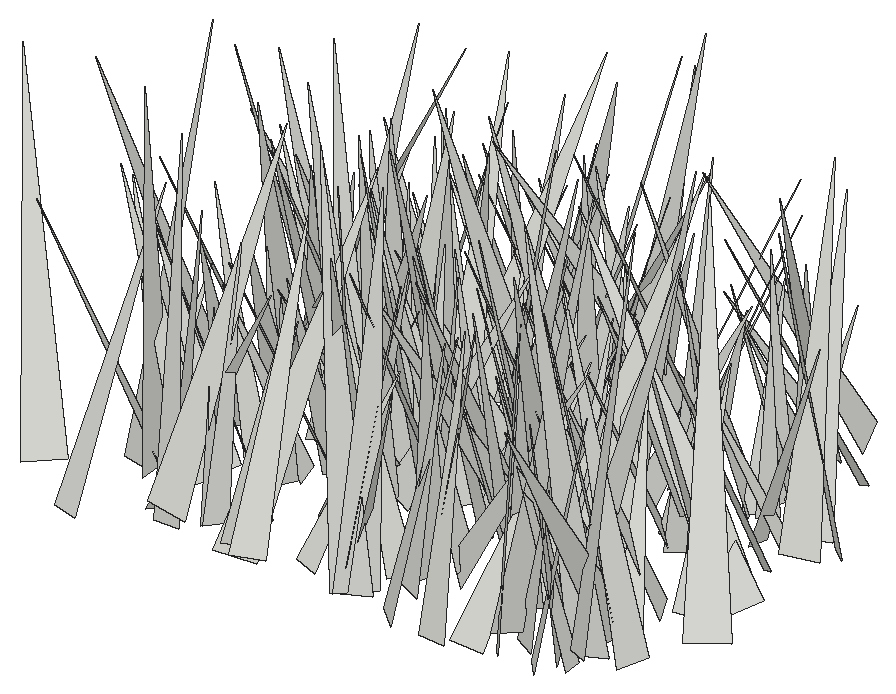
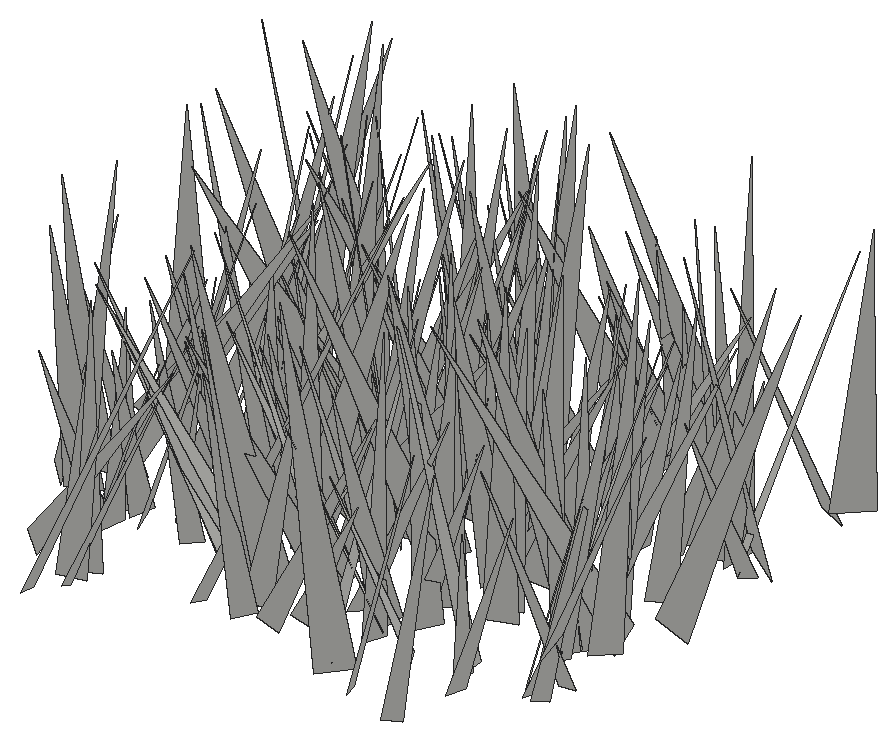
# SketchUp Ruby script. Lengths in inches.
U = 1.inch
M = Sketchup.active_model
def pt(a) = Geom::Point3d.new(a.map { |v| v * U })
def face(e, loops, mat)
  f = e.add_face(loops[0].map { |a| pt(a) })
  loops[1..].each { |l| e.add_face(l.map { |a| pt(a) }).erase! }
  f.material = f.back_material = mat if mat
  f
end
# faces: each face lists its corners as indices into pts; further lists are holes
def faces(e, pts, list, mat = nil) = list.each { |f| face(e, (f[0].is_a?(Array) ? f : [f]).map { |l| l.map { |i| pts[i] } }, mat) }
# xy, xz, yz: faces in a plane at the given z, y or x. An outline is a flat list of corners, or four numbers for a rectangle; further outlines are holes
def ring(l) = l.size == 4 ? [[l[0], l[1]], [l[2], l[1]], [l[2], l[3]], [l[0], l[3]]] : l.each_slice(2).to_a
def flat(e, list, mat, &to3) = list.each { |f| face(e, (f[0].is_a?(Array) ? f : [f]).map { |l| ring(l).map { |u, v| to3.(u, v) } }, mat) }
def xy(e, z, list, mat = nil) = flat(e, list, mat) { |x, y| [x, y, z] }
def xz(e, y, list, mat = nil) = flat(e, list, mat) { |x, z| [x, y, z] }
def yz(e, x, list, mat = nil) = flat(e, list, mat) { |y, z| [x, y, z] }
def lines(e, pts, list) = list.each { |a, b| e.add_line(pt(pts[a]), pt(pts[b])) }
# prism: a flat outline (further loops are holes) pulled along v
def prism(e, loops, v, mat = nil)
  f = face(e, loops, mat); d = Geom::Vector3d.new(v.map { |x| x * U })
  f.pushpull(f.normal.samedirection?(d) ? d.length : -d.length)
end
def box(e, o, s, mat = nil) = prism(e, [[o, [o[0] + s[0], o[1], o[2]], [o[0] + s[0], o[1] + s[1], o[2]], [o[0], o[1] + s[1], o[2]]]], [0, 0, s[2]], mat)
def at(x, y, z, deg = 0) = Geom::Transformation.translation(pt([x, y, z])) * Geom::Transformation.rotation(ORIGIN, Z_AXIS, deg.degrees)
def axes(o, x, y, z) = Geom::Transformation.new([*x, 0, *y, 0, *z, 0, *pt(o).to_a, 1])
def part(name) = M.definitions.add(name)
# library, detail: a bought-in or finely detailed component or shape, given as its bounding box
def library(name, o, s) = part(name).tap { |d| box(d.entities, o, s) }
def detail(e, o, s) = box(e.add_group.entities, o, s)
def put(e, d, t, mat = nil) = e.add_instance(d, t).tap { |i| i.material = mat if mat }
def group(e, t, mat = nil) = e.add_group.tap { |g| g.transformation = t; g.material = mat if mat }.entities
root = M.entities
c1 = part("fur_instance\#9")
p = [[0.8125,0,1.79],[0.67,-0.02,1.48],[0,-0.11,0],[0,0.11,0]]
faces(c1.entities,p,[[0,1,2,3]])
put(root,c1,axes([88.02,156.51,-28.22],[4.64507,-4.79979,0.2726],[-4.36308,-4.36804,-2.56373],[-2.01887,-1.6035,6.16782]))
put(root,c1,axes([77.79,154.35,-28.22],[5.21952,0.68023,0.61562],[0.83808,-4.98198,-1.60081],[-0.37326,-1.674,5.01433]))
put(root,c1,axes([80.74,152.42,-28.22],[3.65147,4.43575,1.22236],[4.5601,-3.69672,-0.20725],[-0.61278,-1.07778,5.74161]))
put(root,c1,axes([81.4,152.85,-27.1],[1.95636,4.4496,1.57567],[4.70552,-1.97342,-0.26957],[-0.3738,-1.55425,4.8532]))
put(root,c1,axes([72.83,152.17,-27.1],[-3.84179,0.25674,0.88435],[-0.00822,3.78425,-1.13434],[0.92083,1.10494,3.67947]))
put(root,c1,axes([82.99,152.11,-28.22],[0.82489,5.68831,1.342],[5.81529,-0.93413,0.38496],[-0.58339,-1.2684,5.73491]))
put(root,c1,axes([87.29,153.95,-28.22],[3.95748,1.9361,2.48086],[2.44941,-4.39763,-0.47534],[-1.97573,-1.57388,4.37997]))
put(root,c1,axes([86.67,151.25,-27.1],[3.82585,4.29132,1.89582],[3.55577,-4.24822,2.44044],[-3.06039,0.42878,5.20545]))
put(root,c1,axes([85.82,153.8125,-28.22],[-0.58036,-3.55618,1.37675],[-3.59236,0.97706,1.00942],[1.27936,1.13031,3.45894]))
put(root,c1,axes([74.38,151.53,-27.1],[-4.08665,1.67614,0.95166],[1.15635,3.91687,-1.93308],[1.54207,1.50482,3.97156]))
put(root,c1,axes([74.78,151.58,-27.1],[2.09645,3.63188,0.13416],[3.39461,-2.01213,1.42535],[-1.29816,0.60366,3.94386]))
put(root,c1,axes([73.05,152.36,-27.1],[-4.76791,1.69378,1.39092],[1.4281,4.92716,-1.10462],[1.66255,0.62512,4.93778]))
put(root,c1,axes([87.03,152.81,-28.22],[3.56693,3.32971,1.1246],[3.34181,-3.70943,0.38354],[-1.08812,-0.47732,4.86445]))
put(root,c1,axes([69.54,153.64,-28.22],[5.28703,-2.12696,0.17156],[-2.11759,-5.17319,1.12251],[0.26309,1.10465,5.58719]))
put(root,c1,axes([81.67,153.56,-28.22],[5.42096,2.25752,1.64956],[2.38588,-5.61122,-0.16143],[-1.45775,-0.7887,5.87002]))
put(root,c1,axes([67.07,151.28,-28.22],[2.05142,5.93925,0.09208],[5.90467,-2.04959,0.65232],[-0.64654,0.12643,6.2496]))
put(root,c1,axes([65.43,152.15,-27.1],[-5.44191,5.3364,0.6963],[5.36336,5.45938,0.07682],[0.44311,-0.54257,7.6214]))
put(root,c1,axes([75.4375,151.14,-27.1],[-4.827,3.94667,0.05385],[3.76525,4.62978,-1.80751],[1.18405,1.36675,5.96733]))
put(root,c1,axes([88.11,153.6875,-28.22],[-5.31837,-1.43549,0.4315],[-1.49067,5.23198,-0.96754],[0.15722,1.04767,5.42306]))
put(root,c1,axes([71.1,151.98,-27.1],[0.33819,7.69063,1.05021],[7.70297,-0.20312,-0.99305],[0.95553,-1.08446,7.63374]))
put(root,c1,axes([67.31,156.37,-28.22],[-4.61159,-4.4726,0.38091],[-4.39573,4.61032,0.9157],[0.90928,-0.396,6.35865]))
put(root,c1,axes([78.73,153.17,-28.22],[-5.99811,4.4385,2.51735],[4.45899,6.44808,-0.74453],[2.48087,-0.8583,7.4245]))
put(root,c1,axes([78.72,152.91,-28.22],[-1.50956,7.97784,1.83345],[8.07703,1.14872,1.65178],[-1.3301,-2.07864,7.94961]))
put(root,c1,axes([78.3125,153.09,-27.1],[3.87453,3.49507,1.24049],[3.40824,-4.0629,0.80191],[-1.46226,-0.20898,5.15601]))
put(root,c1,axes([84.18,155.85,-28.22],[4.37125,-4.19897,0.80164],[-4.19734,-4.43318,-0.33332],[-0.81017,0.31203,6.05212]))
put(root,c1,axes([80.11,155.66,-28.22],[5.51508,-3.1001,1.56666],[-3.03836,-5.73026,-0.64316],[-1.68328,0.18611,6.29389]))
put(root,c1,axes([70.46,152.79,-28.22],[1.63726,6.8228,1.57078],[6.72877,-1.9791,1.58281],[-1.9343,-1.10957,6.83563]))
put(root,c1,axes([76.18,153.52,-28.22],[0.4921,4.23207,0.57816],[4.10963,-0.31046,-1.22532],[1.16432,-0.69285,4.08059]))
put(root,c1,axes([84.22,152.52,-28.22],[-2.22642,5.28944,0.76409],[4.89566,2.35054,-2.00661],[2.14349,0.12554,5.37668]))
put(root,c1,axes([68.81,155.51,-28.22],[3.49606,4.56093,2.47636],[5.16488,-3.35013,-1.12142],[-0.50841,-2.67048,5.63622]))
put(root,c1,axes([88.66,155.73,-28.22],[-5.18557,-4.32883,1.54546],[-4.49087,5.26797,-0.31293],[0.97941,1.23577,6.74766]))
put(root,c1,axes([88.07,154.65,-28.22],[-0.9931,7.68396,2.84346],[8.04191,0.36629,1.81887],[-1.56723,-2.98953,7.53135]))
put(root,c1,axes([79.22,155.12,-28.22],[-4.02277,2.62654,1.01722],[2.78428,3.97624,0.74391],[0.42575,-1.18612,4.74637]))
put(root,c1,axes([88.92,152.92,-27.1],[4.06044,6.49572,1.60929],[6.19974,-4.35997,1.95581],[-2.5194,-0.26008,7.4065]))
put(root,c1,axes([67.64,155.83,-28.22],[7.3985,0.06507,3.2704],[0.28828,-8.06925,-0.49163],[-3.25831,-0.56619,7.38244]))
put(root,c1,axes([85.96,152.64,-27.1],[7.23662,0.86237,3.59764],[-0.54989,-7.56504,2.91946],[-3.65846,2.84288,6.67751]))
put(root,c1,axes([73.79,152.48,-28.22],[-4.61251,5.93847,1.25396],[5.3205,4.71401,-2.75381],[2.92064,0.79104,6.99694]))
put(root,c1,axes([74.57,158.52,-28.22],[5.93446,-4.51627,0.11992],[-4.41947,-5.84426,-1.3935],[-0.93776,-1.03771,7.32616]))
put(root,c1,axes([73.16,155.4,-28.22],[-4.82792,-3.85999,0.34861],[-3.62589,4.30173,-2.58417],[-1.36894,2.21934,5.6152]))
put(root,c1,axes([69.51,155.82,-28.22],[-5.5849,2.54638,0.93821],[2.66389,5.55377,0.78405],[0.51763,-1.10771,6.08773]))
put(root,c1,axes([80.58,156.55,-28.22],[4.45492,4.83666,0.95124],[4.56601,-3.56591,-3.25273],[1.85733,-2.83468,5.71483]))
put(root,c1,axes([89.59,155.23,-28.22],[-6.93734,1.12272,0.61983],[1.08478,6.95591,-0.45824],[0.68406,0.3553,7.01265]))
put(root,c1,axes([85.91,155.92,-28.22],[-6.46812,-3.13785,1.21731],[-3.3431,6.29489,-1.53709],[0.38946,1.92167,7.02282]))
put(root,c1,axes([78.05,159.51,-28.22],[-2.99336,-6.46525,0.18966],[-6.30073,2.9619,1.52434],[1.46161,-0.47255,6.9596]))
put(root,c1,axes([76.05,156.49,-28.22],[-5.53367,-3.1899,2.46645],[-3.58117,5.81278,-0.51687],[1.85312,1.70777,6.3663]))
put(root,c1,axes([82.53,157.33,-28.22],[-3.26871,-2.2439,0.63682],[-2.29753,3.28654,-0.21245],[0.40248,0.53729,3.95909]))
put(root,c1,axes([75.91,156.9,-28.22],[-1.49797,-4.88201,2.75569],[-5.27998,2.18724,1.00478],[1.88406,2.24805,5.00683]))
put(root,c1,axes([71.89,157.7,-28.22],[3.44775,-2.42349,1.09947],[-2.43313,-3.5995,-0.30427],[-1.07797,0.37336,4.2033]))
put(root,c1,axes([82.2,157.69,-28.22],[-1.33118,-5.02308,1.66852],[-5.29255,1.28443,-0.35575],[0.06525,1.70478,5.18429]))
put(root,c1,axes([82.14,159.96,-28.22],[7.22069,-3.00234,1.05262],[-2.62839,-7.10035,-2.22196],[-1.79266,-1.6827,7.49769]))
put(root,c1,axes([88.01,158.9375,-28.22],[-5.06216,-2.56794,0.53616],[-2.44101,5.03776,1.08155],[0.96086,-0.73072,5.57226]))
put(root,c1,axes([85.05,157.84,-28.22],[3.34183,1.38887,0.77255],[1.56239,-3.2005,-1.00466],[-0.29109,-1.23347,3.4767]))
put(root,c1,axes([69.7,157.1875,-28.22],[-4.93751,1.50851,0.32737],[1.53378,4.91815,0.47027],[0.1741,-0.54591,5.14135]))
put(root,c1,axes([68.08,156.23,-28.22],[-3.43494,4.07646,0.13435],[4.04677,3.38429,0.77755],[-0.50915,-0.60283,5.27368]))
put(root,c1,axes([72.09,158.7,-28.22],[-4.26767,-0.91045,0.71231],[-0.70932,4.21373,1.13607],[0.91278,-0.98229,4.21323]))
put(root,c1,axes([81.26,160.03,-28.22],[1.60402,-6.13136,0.73735],[-5.58582,-1.76536,-2.52831],[-2.63361,0.00991,5.81155]))
put(root,c1,axes([80.69,156.97,-28.22],[-7.05105,-1.29004,0.36767],[-1.33665,6.92247,-1.34515],[0.11284,1.38992,7.04075]))
put(root,c1,axes([66.62,156.59,-28.22],[-0.81178,3.59213,0.55552],[3.51446,0.92094,-0.81938],[0.92765,-0.34562,3.5904]))
put(root,c1,axes([86.65,158.11,-28.22],[-4.9499,-5.12629,0.49866],[-4.98162,4.58947,-2.26921],[-1.30806,1.92014,6.75508]))
put(root,c1,axes([86.39,155.75,-28.22],[6.67924,-1.26552,2.75336],[-2.18749,-6.62541,2.26131],[-2.097,2.88046,6.41095]))
put(root,c1,axes([72.96,159.35,-28.22],[1.69834,-4.62751,0.65795],[-4.61755,-1.76962,-0.52709],[-0.72459,0.43091,4.90106]))
put(root,c1,axes([67.92,159.87,-28.22],[3.84252,-3.67557,0.42443],[-3.56655,-3.84235,-0.9854],[-0.98471,-0.42605,5.2253]))
put(root,c1,axes([77.59,158.73,-28.22],[-6.16765,-3.82155,1.90605],[-3.98751,6.35208,-0.16723],[1.52874,1.15063,7.2537]))
put(root,c1,axes([82.94,158.13,-28.22],[-3.53133,-2.30027,1.49102],[-2.55807,3.63918,-0.44418],[0.98523,1.20406,4.19097]))
put(root,c1,axes([73.27,158.94,-28.22],[-3.04212,-3.44962,0.11938],[-3.35963,2.92271,-1.15727],[-0.79185,0.85236,4.45141]))
put(root,c1,axes([66.77,155.62,-28.22],[3.59561,7.30217,1.1805],[7.09033,-3.77639,1.76345],[-2.10771,-0.24675,7.94609]))
put(root,c1,axes([74.57,158.67,-28.22],[1.59006,-7.38899,3.46765],[-7.94346,-2.21328,-1.07372],[-1.87702,3.10714,7.48148]))
put(root,c1,axes([70.87,157.58,-28.22],[-5.26641,1.25593,0.32091],[1.22212,5.2582,-0.5227],[0.43216,0.43524,5.3888]))
put(root,c1,axes([87.9375,157.125,-28.22],[-2.52047,3.62206,0.22803],[3.61381,2.53037,-0.24846],[0.33426,-0.04477,4.40572]))
put(root,c1,axes([74.17,156.91,-28.22],[4.05537,2.07279,0.17475],[1.9711,-3.95155,1.12829],[-0.66463,0.92835,4.41242]))
put(root,c1,axes([75.57,158.63,-28.22],[-6.94561,0.7265,2.56424],[0.79665,7.39636,0.06233],[2.54332,-0.33278,6.98322]))
put(root,c1,axes([84.43,157.01,-28.22],[1.79845,4.31058,0.12569],[4.2592,-1.79684,0.67963],[-0.67534,0.14702,4.621]))
put(root,c1,axes([80.375,160.66,-28.22],[-0.3519,-5.66898,0.64957],[-5.59847,0.21723,-1.13712],[-1.1029,0.70611,5.5649]))
put(root,c1,axes([78.21,158.375,-28.22],[2.39277,4.07076,1.54907],[4.21231,-2.6123,0.35825],[-1.10775,-1.14055,4.7083]))
put(root,c1,axes([75.8,159.96,-28.22],[-1.49578,-4.28811,0.26565],[-3.87905,1.22698,-2.03551],[-1.84701,0.89578,4.0598]))
put(root,c1,axes([84.61,163.27,-28.22],[-3.72735,-5.65721,0.3773],[-4.71825,3.34531,3.54775],[3.14396,-1.68653,5.77153]))
put(root,c1,axes([79.78,159.2,-28.22],[-2.85535,-4.62994,1.75531],[-4.89429,2.33192,-1.81068],[-0.75056,2.40755,5.12941]))
put(root,c1,axes([68.59,161.71,-28.22],[4.17409,-3.35782,0.27535],[-3.2273,-4.11088,-1.20788],[-0.96712,-0.77425,5.2191]))
put(root,c1,axes([77.39,161.27,-28.22],[0.67121,-5.58126,0.90748],[-5.6399,-0.72653,-0.2969],[-0.40679,0.86382,5.61363]))
put(root,c1,axes([76.38,161.85,-28.22],[-1.5232,-7.73744,1.34983],[-7.81047,1.63722,0.57115],[0.82858,1.20901,7.86523]))
put(root,c1,axes([69.56,160.98,-28.22],[-3.27123,-4.88451,0.3113],[-4.82797,3.15879,-1.17003],[-0.80376,0.90546,5.76111]))
put(root,c1,axes([72.42,160.76,-28.22],[5.42547,-4.53511,0.52895],[-4.56014,-5.3411,0.98008],[0.2284,1.09004,7.00303]))
put(root,c1,axes([83.13,162.17,-28.22],[-5.10979,-2.8974,1.28802],[-2.4355,5.15064,1.92434],[2.03034,-1.11347,5.54994]))
put(root,c1,axes([88.51,161.13,-28.22],[-2.84226,-5.05917,1.08036],[-5.16298,2.85167,-0.22901],[0.32566,1.05526,5.79838]))
put(root,c1,axes([83.68,158.89,-28.22],[0.88242,4.55252,0.64978],[4.54635,-0.76413,-0.82042],[0.6916,-0.78549,4.5641]))
put(root,c1,axes([75.6,159.36,-28.22],[1.55014,5.60518,1.20615],[5.3228,-0.94254,-2.46072],[2.13086,-1.72318,5.26933]))
put(root,c1,axes([77.9,160.62,-28.22],[-3.70212,4.89762,1.86065],[5.19102,3.12087,2.11373],[-0.70854,-2.72541,5.76407]))
put(root,c1,axes([66.3125,161.27,-28.22],[-0.79345,-6.87819,1.77521],[-6.83318,0.25089,-2.08208],[-1.94125,1.92821,6.60333]))
put(root,c1,axes([90.73,158.04,-28.22],[-3.36629,7.35026,0.38103],[7.33966,3.3212,0.77612],[-0.54849,-0.66835,8.0471]))
put(root,c1,axes([68.97,160.91,-28.22],[1.04159,-3.44564,1.2731],[-3.64709,-1.12789,-0.06873],[-0.4381,1.19732,3.59897]))
put(root,c1,axes([76.84,159.47,-28.22],[-0.50295,4.78104,0.71911],[4.81704,0.43358,0.48636],[-0.41423,-0.76294,4.78276]))
put(root,c1,axes([84.47,156.71,-28.22],[-6.00676,5.62271,0.83771],[4.81686,5.68135,-3.59416],[3.01902,2.12255,7.40122]))
put(root,c1,axes([88.78,159.125,-28.22],[0.03105,4.61747,0.04613],[4.59439,-0.03553,0.46309],[-0.46341,-0.04278,4.59429]))
put(root,c1,axes([79.21,162.48,-28.22],[3.26712,2.26093,2.86418],[3.20778,-3.61207,-0.80776],[-1.73938,-2.41465,3.89016]))
put(root,c1,axes([90.1,161.23,-28.22],[-2.47066,2.78913,0.64805],[2.82871,2.24449,1.12431],[-0.44456,-1.21919,3.55237]))
put(root,c1,axes([78.18,161.08,-28.22],[-0.19493,4.51759,1.73565],[4.75586,-0.14282,0.90585],[-0.89608,-1.74071,4.43013]))
put(root,c1,axes([80.22,162.13,-28.22],[-2.5232,4.5633,1.53247],[4.25008,1.29942,3.12842],[-2.26029,-2.65076,4.17172]))
put(root,c1,axes([78.11,160.8125,-28.22],[1.55212,3.88569,0.28277],[3.69063,-1.36892,-1.44671],[1.24813,-0.78428,3.92616]))
put(root,c1,axes([79.3,160.83,-28.22],[6.54484,-1.1484,2.12677],[-1.53141,-6.71985,1.08414],[-1.86996,1.48383,6.55579]))
put(root,c1,axes([90.1875,160.7,-28.22],[-3.77529,6.85051,0.02559],[5.94676,3.26269,3.89536],[-3.40091,-1.89957,6.78296]))
put(root,c1,axes([74.28,161.26,-28.22],[-0.09344,5.23116,1.72248],[5.50098,0.0052,0.28262],[-0.26677,-1.725,5.22436]))
put(root,c1,axes([77.83,162.1875,-28.22],[6.04593,4.4435,2.18806],[4.86244,-5.98205,-1.28733],[-0.94282,-2.35709,7.39194]))
put(root,c1,axes([73.28,162.3,-28.22],[-3.32714,-4.87132,0.7615],[-4.7527,2.92423,-2.05917],[-1.31203,1.7603,5.52806]))
put(root,c1,axes([86.41,163.23,-28.22],[-1.00098,-5.50903,0.83943],[-5.47181,0.81017,-1.20786],[-1.05515,1.02481,5.46739]))
put(root,c1,axes([67.07,164.07,-28.22],[6.33398,-2.31725,1.64534],[-1.9481,-6.46653,-1.60778],[-2.06922,-1.00519,6.55011]))
put(root,c1,axes([68.24,164.75,-28.22],[6.05103,1.03829,2.78411],[2.19851,-5.8136,-2.61017],[-1.99898,-3.2509,5.55698]))
put(root,c1,axes([82.19,161.04,-28.22],[0.12612,4.07155,0.3622],[4.08216,-0.1442,0.19951],[-0.2114,-0.35539,4.06861]))
put(root,c1,axes([84.29,161.63,-28.22],[-4.08375,3.22336,1.0157],[3.24667,4.18417,-0.22495],[0.93853,-0.4488,5.19774]))
put(root,c1,axes([71.89,161.6,-28.22],[-1.69454,7.12423,1.83382],[7.32335,1.45532,1.11334],[-0.69716,-2.02889,7.23786]))
put(root,c1,axes([78.29,164.63,-28.22],[-7.9399,0.37328,2.34081],[0.92834,8.01881,1.87016],[2.18103,-2.05426,7.72553]))
put(root,c1,axes([73.05,162.47,-28.22],[-3.27295,5.40819,2.7555],[5.57889,3.91368,-1.05481],[2.39109,-1.7286,6.23283]))
put(root,c1,axes([82.92,163.13,-28.22],[-2.12698,-6.60371,3.80122],[-7.1046,3.14508,1.48842],[2.75369,3.0136,6.77625]))
put(root,c1,axes([67.91,164.45,-28.22],[5.00192,-1.81934,1.03799],[-1.65,-5.07776,-0.94895],[-1.29032,-0.55947,5.23724]))
put(root,c1,axes([78.18,162.01,-28.22],[-1.50833,4.20798,0.27956],[4.21722,1.50618,0.08227],[0.01672,-0.29093,4.46939]))
put(root,c1,axes([71.85,163.7,-28.22],[1.65081,-5.08845,2.41171],[-5.51574,-1.96719,-0.37505],[-1.13372,2.16141,5.33637]))
put(root,c1,axes([89.14,163.42,-28.22],[-5.76145,-5.93812,0.42997],[-5.44241,5.01036,-3.73055],[-2.41379,2.87671,7.38502]))
put(root,c1,axes([69.33,163.87,-28.22],[-5.88104,-3.53705,0.94417],[-3.64814,5.81133,-0.9531],[0.30541,1.30636,6.79625]))
put(root,c1,axes([80.65,164.04,-28.22],[-0.03383,-6.90938,2.82252],[-7.12958,-0.80509,-2.05628],[-2.20801,2.70547,6.5964]))
put(root,c1,axes([71.45,164.54,-28.22],[2.04038,-5.82637,1.87095],[-6.1057,-2.07021,0.21174],[-0.4092,1.83789,6.16967]))
put(root,c1,axes([84.73,163.05,-28.22],[1.48501,3.27806,0.44782],[3.28348,-1.52047,0.24164],[-0.40618,-0.30651,3.59062]))
put(root,c1,axes([71.04,160.99,-28.22],[-6.96616,2.88196,1.8212],[2.05018,6.85162,-3.00033],[2.72382,2.21349,6.91601]))
put(root,c1,axes([68.31,164.7,-28.22],[2.66304,-4.00114,1.09323],[-4.14622,-2.60379,0.57024],[-0.11461,1.22768,4.77239]))
put(root,c1,axes([73.46,164.74,-28.22],[-0.58668,-6.43534,2.37936],[-6.81319,0.82822,0.56013],[0.80964,2.30643,6.43771]))
put(root,c1,axes([69.51,163.74,-28.22],[-4.98087,1.16288,0.32288],[1.15979,4.99131,-0.08543],[0.33384,0.00996,5.1141]))
put(root,c1,axes([79.87,164.93,-28.22],[0.12589,-6.48138,2.39431],[-6.90548,-0.03647,0.26437],[0.23531,2.39734,6.47721]))
put(root,c1,axes([88.42,165.32,-28.22],[-3.57731,-0.93265,0.01118],[-0.92223,3.54345,0.51048],[0.1395,-0.49118,3.66148]))
put(root,c1,axes([75.78,162.1,-28.22],[-5.45003,5.37343,0.92209],[5.18096,5.51046,-1.48977],[1.69756,0.43353,7.50714]))
put(root,c1,axes([87.63,164.76,-28.22],[4.29201,-0.29938,0.77765],[-0.39482,-4.32378,0.51456],[-0.73381,0.57535,4.27156]))
put(root,c1,axes([85.03,165.62,-28.22],[-4.36965,-1.59831,1.51111],[-1.58231,4.61869,0.30967],[1.52785,0.21216,4.64247]))
put(root,c1,axes([82.38,164.87,-28.22],[0.36945,4.73641,1.83647],[4.53767,0.52011,-2.25427],[2.28381,-1.79961,4.18191]))
put(root,c1,axes([68.13,165.61,-28.22],[-6.02827,1.48886,1.73676],[1.72693,6.17226,0.7029],[1.50026,-1.12234,6.1695]))
put(root,c1,axes([73.94,165.24,-28.22],[-4.31803,3.62073,2.04082],[3.93255,4.51165,0.31626],[1.34522,-1.56695,5.62628]))
put(root,c1,axes([73.21,166.41,-28.22],[5.97247,-1.71505,1.0533],[-1.60325,-6.04797,-0.7569],[-1.21673,-0.44932,6.16757]))
put(root,c1,axes([67.22,162.84,-28.22],[7.33228,1.89466,0.16833],[1.78282,-7.07911,2.02191],[-0.66303,1.91751,7.29821]))
put(root,c1,axes([79.54,165.39,-28.22],[-3.1989,2.68909,0.37978],[2.66785,3.00183,1.21655],[-0.50792,-1.16886,3.99802]))
put(root,c1,axes([85.89,166.68,-28.22],[-6.24569,-2.79636,0.92417],[-2.76847,6.31368,0.39421],[1.00464,0.01396,6.83176]))
put(root,c1,axes([85.73,162.44,-28.22],[2.20032,6.76237,0.49836],[6.15454,-2.21163,2.83722],[-2.84601,0.44546,6.52083]))
put(root,c1,axes([75.01,163.21,-28.22],[-0.97355,8.05143,1.14446],[7.84551,1.23329,-2.00251],[2.14086,-0.85824,7.85896]))
put(root,c1,axes([74.04,165.74,-28.22],[-3.83694,1.86592,0.39498],[1.90547,3.78872,0.61201],[0.08273,-0.72368,4.22246]))
put(root,c1,axes([79.88,163.77,-28.22],[4.5765,3.32185,0.66717],[3.07667,-4.544,1.52],[-1.41913,0.86116,5.4469]))
put(root,c1,axes([80.71,170.02,-28.22],[-7.67561,-3.02253,0.64542],[-2.50236,7.09168,3.4516],[1.81396,-3.00659,7.49247]))
put(root,c1,axes([90.4,165.875,-28.22],[2.96491,4.33641,3.25393],[4.46173,-4.05854,1.34327],[-3.07985,-1.70497,5.07846]))
put(root,c1,axes([77.65,166.35,-28.22],[3.19259,1.80159,0.09548],[1.75198,-3.04965,-1.03811],[0.43061,-0.9494,3.51578]))
put(root,c1,axes([66.78,168.14,-28.22],[-4.32761,-0.50237,2.11035],[0.41917,4.42689,1.9134],[2.12844,-1.89326,3.91401]))
put(root,c1,axes([67.3,168.02,-28.22],[-5.22696,-1.19875,0.73288],[-0.94186,5.08442,1.59898],[1.04259,-1.41663,5.11873]))
put(root,c1,axes([86.75,166.43,-28.22],[-2.3678,2.48019,1.72309],[2.76192,2.66404,-0.03926],[1.22155,-1.2159,3.42875]))
put(root,c1,axes([83.5,166.9,-28.22],[1.56073,-4.1385,0.9971],[-4.17951,-1.28812,1.1957],[0.80812,1.33073,4.25833]))
put(root,c1,axes([77.42,165.67,-28.22],[4.89085,0.64493,0.58721],[0.56841,-4.89366,0.64042],[-0.66156,0.56328,4.89144]))
put(root,c1,axes([78.72,166,-28.22],[-2.42701,4.03219,1.90827],[4.11447,2.86278,-0.81615],[1.72373,-1.15601,4.63496]))
put(root,c1,axes([67.6875,167.79,-28.22],[-3.08221,-2.2445,0.63722],[-2.14243,3.14072,0.69983],[0.92405,-0.20483,3.74807]))
put(root,c1,axes([89.44,164.83,-28.22],[-1.40207,7.22786,1.13046],[7.31414,1.36087,0.37039],[-0.15287,-1.17973,7.35327]))
put(root,c1,axes([75.82,167.04,-28.22],[-4.51711,1.79985,0.33219],[1.82954,4.41557,0.95372],[-0.05124,-1.00862,4.76803]))
put(root,c1,axes([76.49,165.22,-28.22],[4.77639,3.07128,1.21309],[2.81816,-4.90311,1.31748],[-1.72115,0.49496,5.52367]))
put(root,c1,axes([70.16,167.68,-28.22],[6.75177,1.95337,0.7466],[2.07523,-6.56983,-1.57805],[-0.25785,-1.72661,6.84922]))
put(root,c1,axes([87.69,167.02,-28.22],[-4.15206,-1.52587,0.16301],[-1.50616,3.96212,-1.27574],[-0.29385,1.25209,4.2356]))
put(root,c1,axes([74.13,168.32,-28.22],[5.48977,-0.87036,1.92832],[-0.64898,-5.79667,-0.76876],[-2.01365,-0.50463,5.50492]))
put(root,c1,axes([82.33,166.64,-28.22],[4.47916,2.33614,0.04477],[2.33654,-4.47877,-0.05982],[-0.01203,-0.07375,5.05142]))
put(root,c1,axes([74.47,170.6875,-28.22],[-3.43989,-5.36661,0.1848],[-4.97328,3.26677,2.29397],[2.02515,-1.09328,5.94736]))
put(root,c1,axes([82.53,166.35,-28.22],[5.67742,2.27779,0.25934],[2.25803,-5.67581,0.41845],[-0.39608,0.29237,6.10297]))
put(root,c1,axes([66.63,166.77,-28.22],[1.35315,4.35582,0.79538],[4.34518,-1.14634,-1.11449],[0.85157,-1.07217,4.42291]))
put(root,c1,axes([86.22,166.3125,-28.22],[-3.56654,2.39752,0.7344],[2.22273,3.6139,-1.00345],[1.16058,0.44646,4.17868]))
put(root,c1,axes([88.96,166.2,-28.22],[-2.49742,5.95651,1.04282],[6.02179,2.55284,-0.16018],[0.55273,-0.89868,6.45689]))
put(root,c1,axes([86.5,167.66,-28.22],[-4.53937,1.16522,1.40638],[1.15678,4.75002,-0.2018],[1.41333,-0.14527,4.6822]))
put(root,c1,axes([77.58,166.38,-28.22],[6.07013,4.91373,1.22638],[4.90353,-6.18107,0.495],[-1.26656,-0.38061,7.79399]))
put(root,c1,axes([81.43,166.21,-28.22],[5.6659,3.07924,0.02777],[3.03508,-5.59401,1.03936],[-0.52039,0.90013,6.36426]))
put(root,c1,axes([77.02,166.875,-28.22],[5.97099,-0.01983,0.33196],[-0.11666,-5.7151,1.75709],[-0.31141,1.76085,5.70664]))
put(root,c1,axes([85.29,171.51,-28.22],[-0.94018,-7.50089,0.47804],[-7.29693,1.02641,1.75419],[1.80188,0.24278,7.35324]))
put(root,c1,axes([78.375,169.01,-28.22],[-2.71564,-2.49022,0.0198],[-2.39499,2.6036,-1.03032],[-0.68234,0.77224,3.53756]))
put(root,c1,axes([74.64,167.34,-28.22],[2.99625,3.60782,0.19235],[3.59342,-3.00177,0.328],[-0.37513,0.06212,4.67828]))
put(root,c1,axes([77.74,169.84,-28.22],[0.12283,-4.44104,1.09952],[-4.1986,-0.54638,-1.73783],[-1.81756,0.96203,4.08875]))
put(root,c1,axes([74.375,167.23,-28.22],[4.91626,-1.03874,2.91243],[-2.03601,-5.20453,1.58061],[-2.3272,2.35896,4.76972]))
put(root,c1,axes([85.59,170.49,-28.22],[-3.49973,-1.74713,0.54329],[-1.50598,3.41664,1.28623],[1.03907,-0.93268,3.69408]))
put(root,c1,axes([86.74,168,-28.22],[3.51726,-1.23078,1.44078],[-1.67757,-3.4351,1.16087],[-0.88116,1.62697,3.54095]))
put(root,c1,axes([78.91,168.98,-28.22],[1.69917,-3.99461,2.49122],[-4.30676,-2.38859,-0.89256],[-1.90128,1.84064,4.24822]))
put(root,c1,axes([78.78,169.88,-28.22],[3.70766,-2.56946,0.56874],[-2.62102,-3.69364,0.39947],[-0.23628,0.65362,4.49325]))
put(root,c1,axes([69.5,169.49,-28.22],[-4.13289,0.76106,0.51137],[0.79822,4.14817,0.27763],[0.45116,-0.36746,4.1932]))
put(root,c1,axes([72.24,168.55,-28.22],[3.48298,2.03603,0.22687],[2.02285,-3.48877,0.25421],[-0.32396,0.10555,4.02641]))
put(root,c1,axes([79.22,167.71,-28.22],[-6.57541,3.25527,2.97746],[2.73361,7.20101,-1.83599],[3.46258,0.49673,7.10365]))
put(root,c1,axes([69.94,168.54,-28.22],[-3.61922,1.27993,0.57976],[1.16278,3.62754,-0.74965],[0.78884,0.52519,3.76496]))
put(root,c1,axes([85.06,170.83,-28.22],[1.74282,-4.6233,0.69197],[-4.67126,-1.6936,0.44965],[0.18179,0.80496,4.92038]))
put(root,c1,axes([76.94,168.91,-28.22],[-1.27036,4.00789,0.19304],[3.62684,1.0603,1.85365],[-1.71652,-0.72583,3.77372]))
put(root,c1,axes([87.95,170.37,-28.22],[-2.89235,-4.23355,0.19447],[-3.82387,2.50545,-2.32964],[-1.82723,1.45817,4.56743]))
put(root,c1,axes([85.08,172.06,-28.22],[-4.08154,-1.42978,0.42723],[-1.12455,3.76494,1.85644],[0.98091,-1.633,3.906]))
put(root,c1,axes([73.78,170.96,-28.22],[4.17452,-5.37379,1.20818],[-5.50555,-4.02647,1.11376],[0.16212,1.6352,6.71296]))
put(root,c1,axes([85.95,173.19,-28.22],[-6.53247,-2.60599,0.49941],[-2.30056,6.22381,2.3844],[1.32211,-2.04617,6.61657]))
put(root,c1,axes([79.9,168.25,-28.22],[2.36714,6.37429,1.14743],[6.22522,-2.57637,1.46983],[-1.78738,-0.5313,6.63886]))
put(root,c1,axes([72.49,171.71,-28.22],[-3.9819,-2.09854,0.99873],[-1.89028,4.07705,1.03024],[1.35209,-0.4803,4.38155]))
put(root,c1,axes([69.99,172.49,-28.22],[4.10212,-1.60455,0.85508],[-1.23063,-4.00368,-1.60913],[-1.3384,-1.23658,4.10033]))
